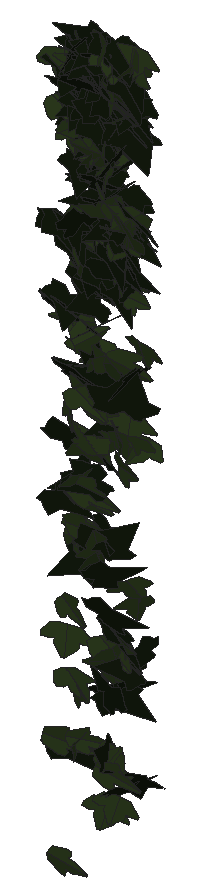
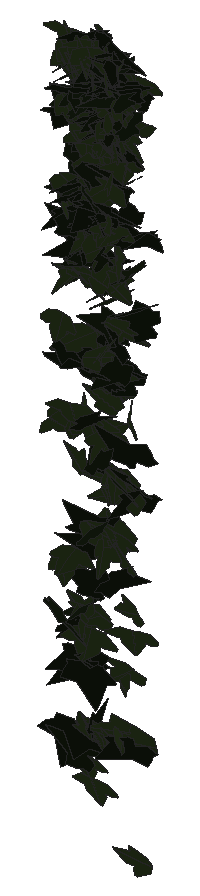
# SketchUp Ruby script. Lengths in millimetres.
U = 1.mm
M = Sketchup.active_model
def pt(a) = Geom::Point3d.new(a.map { |v| v * U })
def face(e, loops, mat)
  f = e.add_face(loops[0].map { |a| pt(a) })
  loops[1..].each { |l| e.add_face(l.map { |a| pt(a) }).erase! }
  f.material = f.back_material = mat if mat
  f
end
# faces: each face lists its corners as indices into pts; further lists are holes
def faces(e, pts, list, mat = nil) = list.each { |f| face(e, (f[0].is_a?(Array) ? f : [f]).map { |l| l.map { |i| pts[i] } }, mat) }
# xy, xz, yz: faces in a plane at the given z, y or x. An outline is a flat list of corners, or four numbers for a rectangle; further outlines are holes
def ring(l) = l.size == 4 ? [[l[0], l[1]], [l[2], l[1]], [l[2], l[3]], [l[0], l[3]]] : l.each_slice(2).to_a
def flat(e, list, mat, &to3) = list.each { |f| face(e, (f[0].is_a?(Array) ? f : [f]).map { |l| ring(l).map { |u, v| to3.(u, v) } }, mat) }
def xy(e, z, list, mat = nil) = flat(e, list, mat) { |x, y| [x, y, z] }
def xz(e, y, list, mat = nil) = flat(e, list, mat) { |x, z| [x, y, z] }
def yz(e, x, list, mat = nil) = flat(e, list, mat) { |y, z| [x, y, z] }
def lines(e, pts, list) = list.each { |a, b| e.add_line(pt(pts[a]), pt(pts[b])) }
# prism: a flat outline (further loops are holes) pulled along v
def prism(e, loops, v, mat = nil)
  f = face(e, loops, mat); d = Geom::Vector3d.new(v.map { |x| x * U })
  f.pushpull(f.normal.samedirection?(d) ? d.length : -d.length)
end
def box(e, o, s, mat = nil) = prism(e, [[o, [o[0] + s[0], o[1], o[2]], [o[0] + s[0], o[1] + s[1], o[2]], [o[0], o[1] + s[1], o[2]]]], [0, 0, s[2]], mat)
def at(x, y, z, deg = 0) = Geom::Transformation.translation(pt([x, y, z])) * Geom::Transformation.rotation(ORIGIN, Z_AXIS, deg.degrees)
def axes(o, x, y, z) = Geom::Transformation.new([*x, 0, *y, 0, *z, 0, *pt(o).to_a, 1])
def part(name) = M.definitions.add(name)
# library, detail: a bought-in or finely detailed component or shape, given as its bounding box
def library(name, o, s) = part(name).tap { |d| box(d.entities, o, s) }
def detail(e, o, s) = box(e.add_group.entities, o, s)
def put(e, d, t, mat = nil) = e.add_instance(d, t).tap { |i| i.material = mat if mat }
def group(e, t, mat = nil) = e.add_group.tap { |g| g.transformation = t; g.material = mat if mat }.entities
root = M.entities
M.materials.add("efeu1").color = [18, 25, 13]
M.materials.add("efeu2").color = [43, 57, 29]
c1 = part("ivyleaf_10")
p = [[0,12.8,-0.8],[-1.5,51.3,-10.9],[-4.9,51,-11.6],[-13.6,26.5,-7.3],[-13.2,15.9,-4.6],[-21.1,19.3,-7.2],
  [-29.5,16.3,-8.3],[-29.2,8.3,-6.2],[-19.7,-9.8,0.5],[-7.6,-13,4],[1,-12.2,5.8],[-0.4,51.1,-11.1],
  [-1.5,51.1,-10.9],[1,-12.4,5.9],[16.9,-12.4,3.5],[35.1,9.1,-5.1],[35,12.9,-6.1],[20.5,16.4,-4.9],
  [15.8,15,-3.8],[15.3,27.6,-7.1],[12.8,31.3,-7.8]]
faces(c1.entities,p,[[0,1,2,3,4,5,6,7,8,9,10],[11,12,0,13,14,15,16,17,18,19,20]],"efeu2")
c2 = part("ivyleaf_9")
p = [[39.1,54.8,31.7],[34.5,51.8,30.2],[-5.3,25.2,17.3],[-17.9,28.3,20.9],[-21.6,21.7,17],[-20.2,4.3,5.3],
  [-22.9,-0.3,2.5],[-17.1,-4,-0.6],[-2,-2.1,-1.2],[-0.7,-15.4,-10.1],[16.6,-22.3,-16.7],[21.1,-15.1,-12.5],
  [32.7,-10.7,-11],[46.1,-1.8,-6.6],[30.8,11.2,3.8]]
faces(c2.entities,p,[[0,1,2,3,4,5,6,7,8,9,10,11,12,13,14]],"efeu1")
put(root,c1,axes([2589.4,948.7,1454],[1.05711,-0.65414,0.12328],[0.16207,-0.08941,-0.85812],[1.25647,0.56189,0.00697]))
put(root,c1,axes([2559.8,940.4,989.2],[1.09543,0.24818,0.51363],[0.85726,0.25001,-0.62555],[-0.66619,0.72979,0.03962]))
put(root,c2,axes([2592.9,949.8,601.2],[0.33946,-0.13445,0.78479],[1.15262,-0.4992,-0.22316],[0.98377,0.63127,-0.00933]))
put(root,c2,axes([2646.9,940.4,994.6],[-1.4492,-0.03775,0.58295],[1.10924,-0.11392,0.75392],[0.07526,0.95219,0.11331]))
put(root,c2,axes([2516.6,947.7,1290.7],[-0.81149,-0.30085,-0.56503],[0.84043,0.35327,-0.52133],[0.88201,-0.61341,-0.02311]))
put(root,c1,axes([2583.6,943.6,901.1],[1.10854,0.01244,0.47439],[-0.90259,-0.01166,0.58259],[0.03236,-0.75112,-0.00119]))
put(root,c2,axes([2593.4,950.9,1531.8],[-1.4661,0.19179,-0.20522],[0.35482,-0.09896,-0.79232],[-0.39985,-0.79104,0.04936]))
put(root,c1,axes([2653.3,946.6,1293],[-1.62255,0.32496,-0.16501],[-0.30627,0.041,0.91218],[0.62235,0.86739,0.0187]))
put(root,c2,axes([2522.4,960.1,1146.6],[-0.49869,-0.74455,0.21268],[-0.03884,-0.21781,-0.78765],[1.47319,-0.25778,0.05123]))
put(root,c1,axes([2593.2,938.4,1440.5],[-0.47083,0.17221,0.81277],[-1.47646,0.25564,-0.29029],[-0.56593,-0.81021,0.08116]))
put(root,c2,axes([2630.2,936.2,455.8],[0.09274,-0.06134,0.83268],[-0.52568,0.78595,0.07406],[-1.49958,-0.27931,0.02553]))
put(root,c1,axes([2603.8,945.2,322.4],[0.34567,0.01122,0.75224],[1.39935,0.16121,-0.17993],[-0.30318,0.75687,0.02717]))
put(root,c1,axes([2536.5,955.9,440.2],[-0.40958,0.17067,0.69672],[1.0441,-0.42948,0.27466],[0.87955,0.5893,-0.0016]))
put(root,c1,axes([2623.2,943.4,548.1],[-0.64734,-0.76932,-0.27925],[0.25553,0.24586,-0.84086],[1.53654,-0.365,0.02219]))
put(root,c1,axes([2661,953.9,1342.1],[-0.93313,-0.3673,0.47625],[-0.55463,-0.39241,-0.60266],[1.0013,-0.55966,0.11001]))
put(root,c2,axes([2529.4,937.4,1548.5],[1.54307,0.19878,0.19434],[0.34725,0.0716,-0.8344],[-0.3992,0.83067,0.02541]))
put(root,c1,axes([2625.9,949.8,273.4],[1.45928,-0.11645,-0.02617],[-0.0484,0.00684,-0.77554],[0.22193,0.76716,0.00294]))
put(root,c1,axes([2567.4,929.7,1094.2],[0.21745,0.11293,-0.94264],[0.76417,0.8546,0.15105],[1.63731,-0.41386,0.05469]))
put(root,c2,axes([2598.9,961.1,341.3],[0.07202,0.05672,0.78925],[-0.69193,-0.70056,0.06778],[1.3376,-0.36545,-0.00743]))
put(root,c1,axes([2600.5,959.9,1398.6],[-0.42325,0.34672,-0.67417],[-0.02194,-0.70404,-0.35828],[-1.44265,-0.09102,0.20324]))
put(root,c1,axes([2531,949.5,469.4],[1.16731,0.0572,0.44802],[0.85032,0.03384,-0.61597],[-0.12592,0.75879,-0.0063]))
put(root,c2,axes([2568.2,954.2,1547.1],[1.11795,-0.58266,0.31966],[0.43255,-0.22478,-0.82737],[1.18857,0.62984,0.00043]))
put(root,c2,axes([2595.8,937.3,671.6],[0.20174,0.06134,0.80519],[1.41982,0.30343,-0.12133],[-0.58831,0.75333,-0.0167]))
put(root,c1,axes([2607.1,950.9,1325.1],[-1.41794,-0.50115,0.12123],[0.19275,0.06665,0.8979],[-0.96219,0.75188,0.00122]))
put(root,c2,axes([2542.6,932.9,1287.9],[0.15445,0.08448,0.90621],[1.30276,0.59395,-0.11667],[-1.14161,0.68923,-0.01053]))
put(root,c1,axes([2598.5,943.2,1633.2],[0.64403,-0.6322,-0.47254],[-0.32319,0.44378,-0.71533],[1.46698,0.37532,0.04986]))
put(root,c2,axes([2627.8,929.5,1434],[-0.39651,0.44217,-0.79802],[-0.85155,0.66384,0.48464],[1.5132,0.48944,0.06362]))
put(root,c1,axes([2548.3,948.6,814.1],[0.37189,0.05851,0.86892],[1.62988,0.14889,-0.20261],[-0.30115,0.87809,-0.02355]))
put(root,c2,axes([2585.6,955.6,1481],[-0.1788,-0.79589,-0.21894],[0.06632,0.21634,-0.80136],[1.5696,-0.0998,0.00892]))
put(root,c2,axes([2512.2,940.4,796.7],[0.13143,-0.29872,-0.75237],[-0.10092,0.75181,-0.30337],[1.53734,0.07489,0.04441]))
put(root,c2,axes([2488.6,953.2,1130],[1.15115,-0.42426,0.40784],[0.63949,-0.23118,-0.7388],[0.91953,0.69191,0.00323]))
put(root,c2,axes([2518.3,956.5,1285.8],[-0.12863,-0.86837,-0.28247],[0.0604,0.28084,-0.87094],[1.73687,-0.07408,0.00937]))
put(root,c1,axes([2514.3,952.9,1578.4],[1.66058,0.0776,0.13545],[0.25676,0.01208,-0.87597],[-0.14947,0.88289,0.00008]))
put(root,c1,axes([2606.7,949.6,1337.1],[-0.70439,0.76913,-0.02259],[-0.05688,0.01068,0.85325],[1.46333,0.37064,0.02229]))
put(root,c1,axes([2499,956.7,126.3],[-0.1359,0.03664,-0.75321],[1.22121,-0.3945,-0.08002],[-0.75396,-0.64559,0.00615]))
put(root,c2,axes([2522.3,956.4,1010.7],[0.82013,-0.42356,0.57102],[0.92252,-0.31345,-0.5983],[0.98989,0.64305,0.08448]))
put(root,c2,axes([2626.3,953.7,1312.2],[-1.34026,0.30749,-0.05921],[0.10585,-0.02059,-0.76841],[-0.58648,-0.7064,-0.00337]))
put(root,c2,axes([2572.7,968.5,1147.6],[-0.79126,-0.29304,0.63154],[-0.46046,-0.62892,-0.4511],[1.24246,-0.4197,0.23502]))
put(root,c2,axes([2652.9,967.4,510.9],[-0.48131,-0.14558,0.80927],[-1.10245,-0.56937,-0.28344],[1.11066,-0.62824,0.06935]))
put(root,c2,axes([2585.5,966.9,1599.5],[-0.99708,-0.5633,0.36182],[-0.47489,-0.26204,-0.76926],[1.18238,-0.58027,-0.00385]))
put(root,c1,axes([2610.3,945.6,1061.2],[-0.99162,0.13899,0.70175],[-1.28382,0.19362,-0.53919],[-0.45336,-0.85231,-0.00805]))
put(root,c1,axes([2520.3,953.7,543.6],[1.47639,0.29292,-0.00672],[-0.01192,-0.00244,-0.8292],[-0.55751,0.77577,-0.00007]))
put(root,c1,axes([2605.5,950.3,1543.8],[0.96733,-0.5984,-0.32039],[-0.27386,0.29617,-0.78144],[1.26248,0.52275,0.07598]))
put(root,c1,axes([2536.3,967.7,339.6],[-0.12673,-0.29974,-0.72216],[-0.04464,-0.72368,0.30253],[-1.48743,0.04726,0.05245]))
put(root,c1,axes([2570.3,965.6,1049.4],[-0.24828,0.33759,0.69621],[0.35891,-0.67087,0.36064],[1.42818,0.22728,0.0304]))
put(root,c2,axes([2618.2,951,1013.8],[-0.50648,0.12962,0.83782],[-1.40171,0.39956,-0.29576],[-0.79912,-0.78301,-0.01223]))
put(root,c1,axes([2581.4,963.2,706.7],[-0.77096,-0.76264,-0.38046],[-0.311,-0.34393,0.86341],[-1.59195,0.43653,0.01558]))
put(root,c1,axes([2599,952.9,548.4],[1.13236,0.15305,0.53597],[0.99632,0.1158,-0.61419],[-0.36432,0.79237,-0.01377]))
put(root,c1,axes([2558.8,936.8,1230.8],[0.20282,-0.01039,-0.84988],[0.07148,0.85575,-0.00575],[1.61603,-0.03655,0.10692]))
put(root,c2,axes([2632.6,946.2,1379.9],[-0.27272,0.76912,-0.04322],[0.01791,-0.04221,-0.78235],[-1.46599,-0.1436,-0.00152]))
put(root,c2,axes([2591.4,947.6,1503.4],[-0.83751,-0.49381,0.58323],[0.73286,0.43805,0.66143],[-1.25629,0.58474,-0.00296]))
put(root,c2,axes([2563.9,945.7,1086.5],[0.54958,-0.37027,-0.64372],[-0.71309,0.52368,-0.4693],[1.22026,0.47278,0.01567]))
put(root,c1,axes([2579.7,954.5,1427],[-0.01852,-0.82209,-0.07048],[0.02031,0.07035,-0.82209],[1.5702,-0.01061,0.0098]))
put(root,c1,axes([2554.2,954.9,1075.3],[-0.00767,0.83102,0.18644],[-0.06892,-0.18644,0.83024],[1.61945,-0.004,0.03622]))
put(root,c1,axes([2613.1,962.4,555],[-0.50256,0.02088,0.74855],[1.27181,-0.35164,0.24554],[0.64318,0.71163,0.09937]))
put(root,c1,axes([2607.2,953.6,1613.7],[1.04996,0.64521,0.02485],[0.04016,0.01465,-0.84888],[-1.22821,0.55205,-0.00652]))
put(root,c1,axes([2619.9,963.5,917.6],[-0.61051,0.40567,0.5683],[0.62046,-0.46603,0.51669],[1.17514,0.45681,0.02243]))
put(root,c2,axes([2602.6,968.1,1245.4],[0.1166,-0.74917,0.31351],[0.0331,-0.31312,-0.75163],[1.54527,0.06324,-0.00756]))
put(root,c2,axes([2582.2,959.2,833.8],[-1.47654,0.09988,0.22816],[-0.42924,0.03492,-0.7822],[-0.20108,-0.80792,-0.0056]))
put(root,c1,axes([2512.3,961.1,589.1],[0.61362,-0.083,0.65377],[1.18266,-0.20407,-0.33236],[0.41765,0.6998,-0.01938]))
put(root,c1,axes([2512.6,968,950.9],[0.5077,-0.48349,0.71737],[0.97392,-0.51709,-0.5388],[1.3275,0.56427,0.12093]))
put(root,c2,axes([2550.3,970.8,1501.4],[-0.74895,-0.6603,0.30634],[-0.16875,-0.30217,-0.7652],[1.37503,-0.39674,0.07295]))
put(root,c1,axes([2533.3,951.6,800.2],[-0.95425,-0.05608,-0.73277],[1.38676,0.07765,-0.50451],[0.18225,-0.88448,0.00217]))
put(root,c1,axes([2551.3,953.8,1470.3],[1.19228,-0.38982,-0.50707],[-0.79667,0.28677,-0.73761],[0.92036,0.75322,0.0184]))
put(root,c1,axes([2646.3,959.8,1624.5],[1.09077,-0.60779,0.08293],[0.19214,-0.01848,-0.8332],[1.15154,0.5788,0.06047]))
put(root,c1,axes([2497.7,950.5,344.7],[0.22169,0.01211,0.80753],[1.33503,0.40282,-0.10722],[-0.76174,0.70951,0.0471]))
put(root,c2,axes([2547.4,974,1192.4],[-0.0954,-0.58493,0.65199],[-0.02385,-0.65251,-0.58636],[1.66688,-0.04281,0.02892]))
put(root,c1,axes([2599.9,956.9,326.2],[1.36954,-0.28767,-0.24903],[0.43926,-0.09352,0.77497],[-0.57569,-0.75571,-0.00111]))
put(root,c1,axes([2542.2,966,1571.4],[-0.8366,-0.46717,0.51575],[-0.4227,-0.48394,-0.62765],[1.25513,-0.47437,0.13239]))
put(root,c2,axes([2633.6,962.5,1347.8],[0.78763,-0.68545,0.07201],[0.09729,-0.05324,-0.80053],[1.30811,0.41668,0.01618]))
put(root,c2,axes([2529.2,969.6,1565.3],[-0.90149,-0.67247,0.08596],[-0.05438,-0.08497,-0.82215],[1.28911,-0.47385,0.02543]))
put(root,c2,axes([2606.4,957.1,1212.1],[-1.32755,-0.34063,-0.20475],[-0.35095,-0.089,0.77626],[-0.67006,0.7215,-0.00091]))
put(root,c2,axes([2581.7,962.5,1519.2],[-1.54719,0.05759,0.06096],[-0.11539,0.00688,-0.81497],[-0.11027,-0.81519,-0.00257]))
put(root,c2,axes([2610.3,967.1,1190.5],[0.20109,-0.80781,0.08287],[0.02861,-0.08161,-0.81468],[1.54523,0.10663,0.0043]))
put(root,c2,axes([2612.9,962.7,1634.4],[-0.37005,-0.76154,-0.32238],[0.18731,0.30751,-0.78577],[1.56269,-0.2172,0.01785]))
put(root,c1,axes([2624.6,959.7,1284.4],[1.42905,-0.1518,-0.07309],[-0.13589,0.01567,-0.76605],[0.29043,0.75425,0.0012]))
put(root,c1,axes([2621.2,968.4,1232.1],[0.80941,-0.56538,0.53829],[0.69995,-0.39559,-0.70607],[1.31052,0.56048,0.04465]))
put(root,c1,axes([2560.3,960.6,958.1],[-0.6076,-0.02982,0.67465],[1.28523,-0.01782,0.31877],[0.00642,0.74616,0.03458]))
put(root,c1,axes([2564,959.8,1018.6],[-1.23279,-0.28277,0.33722],[-0.57095,-0.15534,-0.70649],[0.61283,-0.71356,0.02017]))
put(root,c2,axes([2552.3,970.1,1502.6],[-0.54035,-0.75887,0.05999],[-0.07256,-0.04977,-0.81003],[1.44697,-0.28588,-0.01822]))
put(root,c2,axes([2540,972.3,1591.1],[0.085,-0.73931,0.38794],[0.27248,-0.37596,-0.73296],[1.56546,0.10558,0.10651]))
put(root,c1,axes([2611.9,956.7,513],[-1.61594,-0.21455,-0.05141],[0.09785,0.00638,-0.87573],[0.40834,-0.85059,0.0064]))
put(root,c2,axes([2552.7,940.2,1559.3],[-0.5006,0.65465,-0.57528],[-0.60214,0.48818,0.7002],[1.54548,0.40225,0.08646]))
put(root,c2,axes([2569.9,949.7,1585],[0.09262,0.83979,-0.05518],[-0.00713,-0.05506,-0.8412],[-1.60173,0.04881,0.00056]))
put(root,c2,axes([2635.8,965.8,1518.2],[-0.74273,0.41969,-0.60601],[0.77229,-0.45015,-0.57306],[-1.17125,-0.56295,0.00644]))
put(root,c2,axes([2655.5,967.1,1051],[-0.51948,0.41225,-0.65699],[0.52053,-0.60059,-0.49048],[-1.38134,-0.38135,0.06225]))
put(root,c1,axes([2608.5,960.6,351.8],[1.24929,-0.40807,-0.18808],[-0.3068,0.09692,-0.77291],[0.79823,0.67591,-0.00272]))
put(root,c1,axes([2648.6,962.2,1627.3],[1.59675,-0.02794,0.02503],[0.04764,-0.00038,-0.83945],[0.05317,0.83935,0.00046]))
put(root,c2,axes([2535.1,974.8,1380.3],[-0.31079,-0.71639,0.31664],[-0.08515,-0.31439,-0.73437],[1.48825,-0.16759,0.02411]))
put(root,c2,axes([2590.8,954.5,1624.8],[-0.69859,0.03281,-0.83347],[-1.58392,-0.07533,0.36356],[-0.10621,0.90759,0.0603]))
put(root,c1,axes([2616,952.3,1067.8],[-1.0779,-0.35628,-0.73053],[1.21643,0.35482,-0.66856],[0.95559,-0.85355,0.02701]))
put(root,c1,axes([2648.4,971.4,1318.7],[0.25017,-0.711,0.4615],[0.31434,-0.43658,-0.71965],[1.58232,0.19914,0.07]))
put(root,c2,axes([2560.9,945.9,1098],[-0.10325,0.76908,-0.33056],[-0.04678,0.32965,0.77099],[1.59251,0.05955,0.00122]))
put(root,c2,axes([2615.5,952.8,284.3],[0.57822,0.77459,-0.0565],[-0.02164,0.06509,0.83133],[1.47795,-0.30209,0.03427]))
put(root,c2,axes([2640.7,963.6,1481],[-0.57417,-0.59253,-0.4913],[0.46639,0.42629,-0.66461],[1.38871,-0.38816,0.02008]))
put(root,c2,axes([2565.8,970.5,1601.1],[-1.47974,-0.33646,-0.01402],[0.02487,0.0051,-0.84718],[0.64042,-0.77761,0.00051]))
put(root,c2,axes([2605.6,967.9,572.9],[0.59861,-0.81616,-0.00549],[0.01829,0.00959,-0.87458],[1.55325,0.31443,0.01241]))
put(root,c1,axes([2553.1,963.8,1109.9],[-0.3807,0.06176,0.72495],[-1.32621,-0.23253,-0.17246],[0.39831,-0.71519,0.11868]))
put(root,c2,axes([2637.8,952.1,323.3],[1.32774,0.51598,-0.17397],[-0.26717,-0.10277,-0.86772],[-1.0013,0.71162,0.00083]))
put(root,c1,axes([2505.3,954,1493.7],[0.65637,0.63738,0.44975],[0.43883,0.38648,-0.72452],[-1.41831,0.41455,-0.01604]))
put(root,c1,axes([2550.9,958.5,831.4],[-0.62722,-0.7796,-0.26398],[0.18052,0.24649,-0.84636],[1.55606,-0.34284,-0.00822]))
put(root,c2,axes([2627.7,971.5,1563.7],[0.05996,-0.83531,-0.00958],[0.0003,0.00959,-0.8359],[1.58987,0.0315,0.00052]))
put(root,c1,axes([2541.6,953.1,356.4],[0.09529,-0.00593,0.74554],[0.92463,0.56705,-0.02811],[-1.07633,0.4866,0.04185]))
put(root,c2,axes([2547.5,970.3,1608.7],[-0.46379,0.43028,-0.67795],[0.58884,-0.60347,-0.49422],[-1.41022,-0.39349,0.0166]))
put(root,c1,axes([2535.5,970.8,1222],[0.8024,-0.56845,0.36887],[0.48369,-0.27008,-0.7067],[1.19556,0.49079,0.03834]))
put(root,c2,axes([2559,951,1593.2],[1.37414,0.33888,0.21192],[0.32113,0.13824,-0.79591],[-0.68959,0.73967,0.05166]))
put(root,c2,axes([2601,955.6,1237.6],[0.06205,-0.15185,-0.83319],[0.77046,0.73517,-0.11815],[1.41577,-0.39343,0.10081]))
put(root,c2,axes([2555.9,954.9,1371.4],[1.51903,0.12183,0.11698],[0.21395,0.03855,-0.80712],[-0.23992,0.80575,0.02093]))
put(root,c2,axes([2632.1,974.4,1584.1],[0.15452,-0.8197,0.15461],[-0.00915,-0.15579,-0.82348],[1.58754,0.07889,-0.0198]))
put(root,c1,axes([2593.1,965.7,247.3],[1.52303,-0.1316,-0.0261],[-0.04789,0.00785,-0.81099],[0.25081,0.80064,0.00366]))
put(root,c2,axes([2591.6,977.1,1553.5],[-1.27297,-0.45882,0.18135],[-0.1787,-0.18154,-0.80561],[0.9218,-0.66881,0.09426]))
put(root,c2,axes([2515.5,959.1,339.6],[-0.24088,-0.23034,-0.74412],[0.71715,0.64169,-0.26273],[1.2975,-0.39744,0.00707]))
put(root,c2,axes([2611,976.5,1285.1],[0.31866,-0.77195,0.31509],[0.18717,-0.30085,-0.78933],[1.57578,0.19185,0.03004]))
put(root,c1,axes([2602.1,966.4,914.3],[-1.20907,-0.46939,0.21211],[-0.31306,-0.13428,-0.78981],[0.92898,-0.65616,0.0099]))
put(root,c2,axes([2588.3,957.9,715],[-0.73076,0.00007,0.79183],[1.50668,0.01836,0.38388],[-0.03139,0.87982,-0.00808]))
put(root,c2,axes([2581.8,976.6,1464.1],[-0.12135,-0.80231,0.12393],[-0.01763,-0.12358,-0.80484],[1.54497,-0.06443,0.00055]))
put(root,c1,axes([2657,964.1,639.9],[-0.68849,-0.70482,-0.10935],[0.10291,0.09516,-0.79222],[1.35355,-0.36574,0.00461]))
put(root,c2,axes([2587.4,969.5,1456.4],[-1.29343,0.3304,-0.2947],[0.45667,-0.17886,-0.75387],[-0.70813,-0.71884,0.05212]))
put(root,c1,axes([2619.2,958.5,1531.3],[0.22143,0.17729,-0.84393],[-1.4366,0.43271,-0.01316],[0.79361,0.73384,0.21165]))
put(root,c1,axes([2529.9,979.7,1598.2],[-0.07694,-0.18623,0.80476],[0.94309,-0.65011,-0.12555],[1.2578,0.47606,0.14337]))
put(root,c1,axes([2564.3,959.6,891.2],[-1.12028,-0.52168,-0.42239],[0.58315,0.29103,-0.78643],[1.13664,-0.66348,-0.01284]))
put(root,c2,axes([2508.5,965.5,878.6],[-0.32979,0.05557,0.77942],[1.32603,-0.35045,0.17988],[0.67327,0.71743,0.0275]))
put(root,c1,axes([2610.3,969.3,1586.4],[0.35197,-0.82253,0.03934],[0.03306,-0.03641,-0.84302],[1.56688,0.18553,0.00895]))
put(root,c1,axes([2553.9,973.5,1576.3],[0.1351,-0.78043,0.27256],[0.21996,-0.2615,-0.77888],[1.55784,0.1046,0.08634]))
put(root,c2,axes([2632,978.9,1516.2],[0.19625,-0.68691,0.42719],[0.39378,-0.39393,-0.68336],[1.48831,0.1948,0.12448]))
put(root,c1,axes([2653.2,968.3,1600.1],[-0.18734,-0.84393,-0.00061],[0.0049,0.00031,-0.84964],[1.60615,-0.09843,0.00252]))
put(root,c2,axes([2584.4,969.7,1546.9],[0.90248,-0.67063,-0.05659],[0.02127,0.07706,-0.8196],[1.2807,0.4713,0.05349]))
put(root,c2,axes([2632.3,961.1,1298.3],[0.16079,-0.46343,-0.66386],[0.0604,0.66885,-0.46288],[1.53968,0.02216,0.08749]))
put(root,c1,axes([2610.1,977.8,1287.7],[0.33337,-0.29501,0.7157],[1.12007,-0.42596,-0.31961],[0.95712,0.60123,0.12474]))
put(root,c2,axes([2535.9,963.7,1196.6],[0.84795,-0.55438,-0.39868],[-0.21015,0.41128,-0.6953],[1.2825,0.43393,0.14966]))
put(root,c1,axes([2636.8,966.3,924.3],[-1.54639,-0.26571,0.03952],[-0.06455,-0.02343,-0.85478],[0.50718,-0.81314,0.01171]))
put(root,c1,axes([2540.6,971.5,1429.4],[-0.53539,-0.02452,-0.75855],[1.33919,-0.31156,-0.25088],[-0.54125,-0.74664,0.1296]))
put(root,c2,axes([2537.1,975.1,1091.5],[-0.23955,-0.08121,-0.76685],[1.46731,-0.02924,-0.12345],[-0.0302,-0.77656,0.08484]))
put(root,c2,axes([2616.7,981.8,1218],[-0.14062,-0.11055,0.81585],[0.22122,-0.81233,-0.09954],[1.55123,0.10583,0.08815]))
put(root,c2,axes([2586.9,974.7,1012.9],[-1.436,-0.03471,-0.10678],[0.20288,0.00634,-0.75531],[0.06709,-0.76201,-0.00142]))
put(root,c2,axes([2538.3,970.6,1547.5],[-0.52608,-0.1586,0.77641],[1.41573,-0.33539,0.19633],[0.5199,0.75282,0.25103]))
put(root,c2,axes([2636.1,967.6,1199.9],[-1.03,0.53367,-0.0592],[0.08374,-0.0397,-0.76006],[-1.01848,-0.54297,-0.00262]))
put(root,c2,axes([2586.2,973.5,1247.9],[-0.29976,-0.10615,-0.86435],[1.60582,0.19879,-0.17816],[0.41018,-0.85579,0.06582]))
put(root,c2,axes([2613,958.6,461.2],[-0.01011,-0.24572,-0.8413],[0.06754,0.84057,-0.24573],[1.66669,-0.03555,0.00485]))
put(root,c2,axes([2589.5,980.2,1497.4],[-0.29144,-0.81155,0.03216],[-0.01228,-0.03151,-0.82587],[1.54571,-0.15327,-0.0005]))
put(root,c1,axes([2598.5,982.8,1398.3],[0.15589,0.3062,0.83194],[-0.48751,-0.79167,0.31659],[1.61521,-0.2685,0.01526]))
put(root,c2,axes([2595.1,977.4,1396.1],[-1.45595,-0.07871,0.18196],[-0.3355,-0.06188,-0.76787],[0.17267,-0.7839,0.04235]))
put(root,c2,axes([2506.1,980.3,1230.9],[0.24122,-0.77791,0.17103],[0.10669,-0.16404,-0.78766],[1.51212,0.13567,0.02829]))
put(root,c1,axes([2640.2,973.3,1591.8],[-0.95314,-0.66665,0.09852],[0.08234,-0.1543,-0.82417],[1.2799,-0.48653,0.12639]))
put(root,c2,axes([2633.8,981.2,1533],[-1.12746,-0.56296,-0.10351],[0.26212,0.0044,-0.81215],[1.05737,-0.60136,0.09096]))
put(root,c1,axes([2614.4,983.1,1476.5],[-0.04941,-0.61158,0.53138],[0.11287,-0.53166,-0.60901],[1.5378,0.01937,0.06177]))
put(root,c2,axes([2593.3,973.9,1572.2],[-1.50329,0.28737,0.03998],[-0.0862,-0.0076,-0.84022],[-0.54542,-0.79085,0.0226]))
put(root,c1,axes([2645.1,975,1504.4],[-0.44311,-0.78505,0.10537],[-0.02112,-0.10659,-0.81862],[1.50737,-0.23227,0.01951]))
put(root,c1,axes([2581.2,986.3,1051.8],[-0.30461,-0.02137,0.78363],[-0.23463,-0.78916,-0.0467],[1.4734,-0.13009,0.15457]))
put(root,c1,axes([2524.6,971.5,725.8],[-0.25938,-0.0007,0.85387],[1.60137,0.14707,0.13442],[-0.27661,0.85208,-0.0225]))
put(root,c1,axes([2601.8,963.3,1464.3],[-1.0237,0.34717,0.51128],[-0.78225,0.30521,-0.63966],[-0.87836,-0.67644,-0.02621]))
put(root,c2,axes([2553.1,976.8,1563.7],[0.10543,-0.78877,-0.26566],[-0.03145,0.26515,-0.79071],[1.58373,0.05777,0.00198]))
put(root,c1,axes([2630.9,974.7,1586],[1.5075,-0.25243,-0.08969],[-0.15841,0.0342,-0.8313],[0.48461,0.79641,0.00727]))
put(root,c1,axes([2595.8,974,1606.3],[-1.17945,-0.55124,0.12887],[-0.17648,-0.08965,-0.82939],[1.06286,-0.6266,0.00529]))
put(root,c2,axes([2537.3,979.1,1458.1],[-1.1446,-0.14342,-0.53726],[1.00812,0.09306,-0.61779],[0.32204,-0.80105,0.02442]))
put(root,c1,axes([2531.9,970.1,1491.7],[0.42552,0.77697,0.06202],[-0.0584,0.07325,-0.80698],[-1.48229,0.22016,0.0496]))
put(root,c2,axes([2573.2,973.6,1391.2],[0.79164,0.67466,0.34934],[-0.32532,-0.30496,0.79247],[1.40887,-0.44951,-0.0133]))
put(root,c2,axes([2601,978.5,1511.4],[0.68878,-0.74791,-0.03448],[0.03849,0.04805,-0.82995],[1.42442,0.36035,0.0391]))
put(root,c2,axes([2531.9,969.2,1049.8],[1.50442,-0.33972,-0.29967],[-0.5273,0.11427,-0.86037],[0.6821,0.83761,-0.00417]))
put(root,c2,axes([2595.8,976.2,1355],[-1.05654,0.56396,-0.37891],[0.45785,-0.29445,-0.79071],[-1.20932,-0.60419,0.03168]))
put(root,c1,axes([2582,988.2,1251.2],[-0.23321,-0.1424,-0.78255],[-0.76674,-0.67159,0.1853],[-1.30526,0.41995,0.03097]))
put(root,c1,axes([2527.5,978.1,1536.1],[-0.26881,-0.81188,0.10003],[-0.05188,-0.09678,-0.82401],[1.55598,-0.14349,-0.01019]))
put(root,c2,axes([2543.3,961.6,818.1],[-1.05472,0.52698,-0.25199],[-0.37137,0.16039,0.76454],[1.04786,0.58728,0.01732]))
put(root,c2,axes([2673.9,972.5,552.5],[-1.03249,0.62115,-0.0616],[0.07614,-0.04685,-0.82471],[-1.18553,-0.54398,0.00068]))
put(root,c1,axes([2635,969.7,661.8],[-0.95935,-0.50077,-0.37122],[0.50005,0.26224,-0.71054],[1.07584,-0.56844,-0.00076]))
put(root,c1,axes([2535.8,978,731.3],[1.37498,-0.22511,0.02698],[0.04942,-0.00737,-0.75672],[0.42866,0.72292,0.00069]))
put(root,c1,axes([2574.2,978.1,1519.6],[1.21959,-0.52438,0.07588],[0.25227,0.04337,-0.81971],[0.97633,0.64383,0.11702]))
put(root,c1,axes([2553.5,987.7,1212.4],[-0.50979,-0.50231,-0.56287],[-0.52283,-0.49135,0.56921],[-1.33723,0.3836,-0.00796]))
put(root,c2,axes([2620.4,984.3,1360.7],[-0.14913,-0.80406,-0.11492],[0.04449,0.11317,-0.80778],[1.5452,-0.08086,0.01217]))
put(root,c1,axes([2568.8,968,694.2],[-0.24192,-0.77879,-0.53764],[0.17614,0.52963,-0.78908],[1.79245,-0.15716,0.00498]))
put(root,c2,axes([2600.9,992.7,926.7],[-0.60563,-0.38007,0.62949],[-0.78631,-0.47499,-0.49564],[1.15768,-0.52144,-0.00733]))
put(root,c1,axes([2590.7,969.7,1582.1],[0.26156,-0.66064,-0.502],[-0.01694,0.50763,-0.6705],[1.57905,0.11488,0.07596]))
put(root,c2,axes([2580.1,974.9,1469.6],[-1.04537,0.60141,-0.01408],[0.02026,-0.00935,-0.81448],[-1.14474,-0.54937,-0.00156]))
put(root,c1,axes([2516.2,982.6,1432.5],[-0.58297,0.64826,-0.3505],[-0.02646,-0.38458,-0.69916],[-1.40231,-0.26224,0.1589]))
put(root,c2,axes([2623.4,966.1,1409.2],[-0.12819,0.75977,0.21306],[-0.00122,0.21378,-0.76255],[-1.50178,-0.06503,-0.01757]))
put(root,c1,axes([2555.7,980.7,1487.5],[-0.4122,-0.79568,0.03401],[0.01898,-0.03795,-0.8244],[1.5156,-0.21593,0.01957]))
put(root,c2,axes([2590.4,988.1,1291.6],[-1.16227,-0.44917,-0.07114],[0.13177,0.02589,-0.75783],[0.85544,-0.61428,0.02008]))
put(root,c2,axes([2543.9,974.7,1518.9],[1.44548,-0.24942,-0.17916],[-0.3108,0.07673,-0.79912],[0.49498,0.77656,0.02141]))
put(root,c2,axes([2500.5,980.6,1511.6],[1.13161,-0.57068,0.06103],[0.20731,0.02594,-0.81878],[1.07246,0.59714,0.09388]))
put(root,c1,axes([2538.7,982.6,1458.5],[0.64373,-0.71561,0.13946],[0.46596,-0.03333,-0.76479],[1.30699,0.36434,0.20396]))
put(root,c2,axes([2591.5,985.3,1329.9],[-1.24443,-0.00067,0.41071],[-0.78118,-0.02625,-0.6535],[0.02766,-0.77171,0.02187]))
put(root,c1,axes([2535.4,981.5,1511.4],[-0.48732,-0.78178,0.04635],[-0.0138,-0.0464,-0.82261],[1.49043,-0.25604,0.00754]))
put(root,c1,axes([2531.9,980.2,1479.2],[0.74881,-0.72155,-0.09482],[0.03043,0.11633,-0.81892],[1.38472,0.38763,0.06927]))
put(root,c1,axes([2656.5,975.9,1095.1],[-1.33709,0.31466,0.07675],[-0.13413,0.03041,-0.76979],[-0.60165,-0.70607,0.00105]))
put(root,c1,axes([2657.4,988.5,911.2],[0.61312,0.45864,-0.58428],[-0.65676,-0.47155,-0.56042],[-1.25184,0.47202,0.00785]))
put(root,c2,axes([2562.1,995.2,860],[-0.17694,-0.36147,0.73067],[0.21666,-0.73396,-0.34861],[1.53627,0.06188,0.13332]))
put(root,c1,axes([2547,991.7,819.9],[0.28543,-0.35752,0.68886],[0.9228,-0.50468,-0.36749],[1.15337,0.49227,0.12355]))
put(root,c1,axes([2543.1,979.9,1301.7],[-1.06248,-0.46717,-0.23901],[0.59085,-0.01268,-0.70034],[0.80519,-0.60714,0.19854]))
put(root,c2,axes([2530.3,998,661],[0.02609,-0.25941,-0.85154],[0.34645,-0.83282,0.25664],[-1.65838,-0.17807,0.04022]))
put(root,c1,axes([2590.2,969.9,1266.3],[0.37183,0.55454,0.53094],[0.30041,0.50714,-0.58777],[-1.42994,0.25074,0.01458]))
put(root,c2,axes([2518.4,976.5,1553.6],[1.34523,-0.4366,-0.08092],[0.16065,0.28147,-0.78129],[0.82967,0.65339,0.28249]))
put(root,c2,axes([2572.8,971.8,1328.9],[1.34022,0.3322,0.01886],[0.03312,0.00732,-0.77862],[-0.6324,0.70441,-0.00081]))
put(root,c2,axes([2557.1,978.8,1486],[1.42666,-0.31422,-0.06319],[-0.11654,0.01738,-0.81277],[0.59876,0.75207,-0.00762]))
put(root,c2,axes([2622,964.6,471.2],[-0.07644,0.37404,-0.69863],[-0.32092,0.67948,0.37347],[1.47367,0.16737,0.04509]))
put(root,c1,axes([2637.7,967.8,1180.2],[-0.05045,0.4851,0.63075],[-0.04227,0.6304,-0.48577],[-1.51382,-0.03377,-0.00746]))
put(root,c1,axes([2556.8,980.1,1465.9],[0.73783,0.70478,0.03202],[0.03624,0.02608,-0.80436],[-1.34223,0.38813,-0.00411]))
put(root,c1,axes([2535.1,976.9,1258.3],[0.2462,-0.71454,-0.36284],[0.01392,0.36857,-0.72323],[1.52514,0.11198,0.06518]))
put(root,c1,axes([2592.4,984.5,1203.3],[-0.37533,-0.15667,-0.71313],[1.34449,-0.22763,-0.14535],[-0.3512,-0.70401,0.20569]))
put(root,c1,axes([2498.5,991.4,693.3],[0.43695,-0.41364,-0.62472],[0.74584,-0.49059,0.46886],[-1.21537,-0.44978,0.06313]))
put(root,c1,axes([2592.3,985.4,1460.1],[-1.301,-0.44398,0.00443],[0.24202,-0.20357,-0.77899],[0.80963,-0.65259,0.23998]))
put(root,c2,axes([2589,967.5,1294],[-0.08859,0.20816,0.79895],[-0.12355,0.79682,-0.21138],[-1.56646,-0.07462,-0.02851]))
put(root,c2,axes([2608,992.9,1289.6],[0.31056,-0.5104,0.56169],[0.70472,-0.44797,-0.51463],[1.26085,0.3761,0.14929]))
put(root,c1,axes([2601.4,991.3,847.8],[-0.46262,0.1456,0.75017],[1.23706,-0.37455,0.28331],[0.76477,0.69394,-0.00449]))
put(root,c1,axes([2551.8,987.7,1208.7],[-0.97461,-0.35145,0.50491],[-0.75805,-0.31126,-0.62062],[0.89229,-0.6483,0.02425]))
put(root,c1,axes([2546.5,981.4,1403.3],[-0.47605,0.76244,-0.04402],[-0.20664,-0.08136,-0.7921],[-1.43874,-0.24059,0.12833]))
put(root,c2,axes([2620.5,991.9,1344.8],[-0.14162,-0.79708,-0.0449],[-0.00466,0.04532,-0.80052],[1.5194,-0.07416,-0.00664]))
put(root,c1,axes([2624.1,984.5,945.7],[1.40047,0.25516,-0.0371],[-0.06641,-0.0126,-0.77883],[-0.48621,0.73668,-0.00047]))
put(root,c2,axes([2569.6,981.6,1246.7],[1.3061,-0.32844,0.01237],[0.02981,0.00408,-0.76074],[0.62482,0.68636,0.01044]))
put(root,c1,axes([2562.5,980,1313.9],[-1.06086,0.54017,0.0108],[-0.01659,0.00652,-0.7762],[-1.02813,-0.55747,0.00139]))
put(root,c2,axes([2594.2,976.3,461.3],[0.51841,0.73506,-0.23254],[-0.17215,-0.21445,-0.78384],[-1.45716,0.28685,0.00987]))
put(root,c1,axes([2556.2,981.2,1376.1],[-1.31198,-0.16399,-0.41324],[0.79138,0.03205,-0.70636],[0.29949,-0.80309,0.0562]))
put(root,c1,axes([2512.5,983.2,1432.8],[0.93552,0.62875,0.00723],[0.00199,0.00836,-0.79808],[-1.19671,0.49153,0.00433]))
put(root,c2,axes([2572.2,999.7,727.2],[-0.13348,-0.59841,0.53102],[0.01436,-0.53353,-0.60024],[1.52259,-0.04743,0.05221]))
